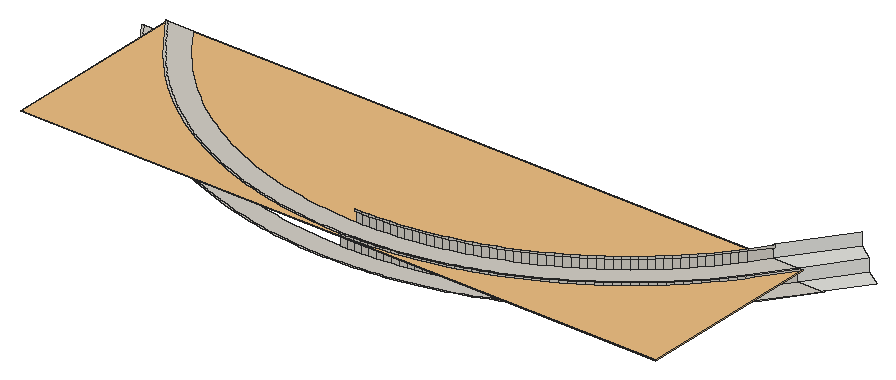
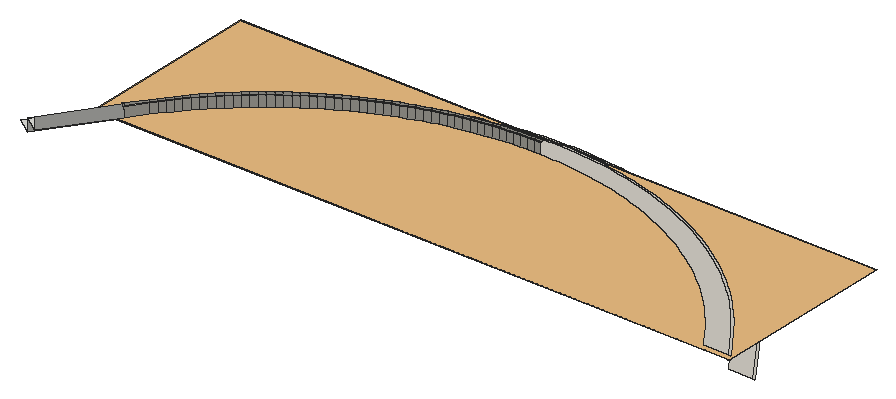
# SketchUp Ruby script. Lengths in inches.
U = 1.inch
M = Sketchup.active_model
def pt(a) = Geom::Point3d.new(a.map { |v| v * U })
def face(e, loops, mat)
  f = e.add_face(loops[0].map { |a| pt(a) })
  loops[1..].each { |l| e.add_face(l.map { |a| pt(a) }).erase! }
  f.material = f.back_material = mat if mat
  f
end
# faces: each face lists its corners as indices into pts; further lists are holes
def faces(e, pts, list, mat = nil) = list.each { |f| face(e, (f[0].is_a?(Array) ? f : [f]).map { |l| l.map { |i| pts[i] } }, mat) }
# xy, xz, yz: faces in a plane at the given z, y or x. An outline is a flat list of corners, or four numbers for a rectangle; further outlines are holes
def ring(l) = l.size == 4 ? [[l[0], l[1]], [l[2], l[1]], [l[2], l[3]], [l[0], l[3]]] : l.each_slice(2).to_a
def flat(e, list, mat, &to3) = list.each { |f| face(e, (f[0].is_a?(Array) ? f : [f]).map { |l| ring(l).map { |u, v| to3.(u, v) } }, mat) }
def xy(e, z, list, mat = nil) = flat(e, list, mat) { |x, y| [x, y, z] }
def xz(e, y, list, mat = nil) = flat(e, list, mat) { |x, z| [x, y, z] }
def yz(e, x, list, mat = nil) = flat(e, list, mat) { |y, z| [x, y, z] }
def lines(e, pts, list) = list.each { |a, b| e.add_line(pt(pts[a]), pt(pts[b])) }
# prism: a flat outline (further loops are holes) pulled along v
def prism(e, loops, v, mat = nil)
  f = face(e, loops, mat); d = Geom::Vector3d.new(v.map { |x| x * U })
  f.pushpull(f.normal.samedirection?(d) ? d.length : -d.length)
end
def box(e, o, s, mat = nil) = prism(e, [[o, [o[0] + s[0], o[1], o[2]], [o[0] + s[0], o[1] + s[1], o[2]], [o[0], o[1] + s[1], o[2]]]], [0, 0, s[2]], mat)
def at(x, y, z, deg = 0) = Geom::Transformation.translation(pt([x, y, z])) * Geom::Transformation.rotation(ORIGIN, Z_AXIS, deg.degrees)
def axes(o, x, y, z) = Geom::Transformation.new([*x, 0, *y, 0, *z, 0, *pt(o).to_a, 1])
def part(name) = M.definitions.add(name)
# library, detail: a bought-in or finely detailed component or shape, given as its bounding box
def library(name, o, s) = part(name).tap { |d| box(d.entities, o, s) }
def detail(e, o, s) = box(e.add_group.entities, o, s)
def put(e, d, t, mat = nil) = e.add_instance(d, t).tap { |i| i.material = mat if mat }
def group(e, t, mat = nil) = e.add_group.tap { |g| g.transformation = t; g.material = mat if mat }.entities
root = M.entities
M.materials.add("Arta-Ceramic-Moonstone-White-24x24-4K").color = [209, 205, 196]
c1 = library("Mesh Light\#6",[-0.5,-0.5,-0.1],[1,1,0.2])
xy(root,18,[[1176.72,194.875,1188.72,194.875,1189.08,195.38,1200.97,212,1193.03,217.67]])
xy(root,18,[[1024.28,97.97,1027.87,98,1031.45,98.11,1035.04,98.28,1038.61,98.52,1042.1875,98.83,1045.76,99.21,1049.3125,99.65,1052.86,100.17,1056.4,100.75,1059.93,101.4,1063.45,102.12,1066.95,102.9,1070.43,103.76,1073.9,104.67,1077.35,105.66,1080.78,106.71,1084.18,107.83,1087.57,109.01,1090.93,110.26,1094.27,111.57,1097.59,112.94,1100.87,114.38,1104.13,115.88,1107.36,117.44,1110.56,119.07,1113.72,120.75,1116.86,122.5,1119.95,124.31,1123.02,126.17,1126.05,128.09,1129.04,130.08,1131.99,132.11,1134.9,134.21,1137.77,136.36,1140.6,138.5625,1143.39,140.82,1146.13,143.13,1148.83,145.5,1151.48,147.91,1154.08,150.38,1156.64,152.89,1159.15,155.46,1161.61,158.07,1164.02,160.73,1166.375,163.43,1168.68,166.18,1170.93,168.97,1173.13,171.81,1175.27,174.68,1189.74,194.91,1189.08,195.38,1188.72,194.875,1174.61,175.16,1172.48,172.3,1170.29,169.48,1168.05,166.7,1165.76,163.96,1163.41,161.27,1161.01,158.62,1158.5625,156.02,1156.07,153.47,1153.52,150.96,1150.93,148.51,1148.29,146.1,1145.6,143.75,1142.87,141.45,1140.09,139.2,1137.28,137.01,1134.42,134.86,1131.52,132.78,1128.58,130.75,1125.6,128.78,1122.59,126.86,1119.54,125,1116.45,123.21,1113.33,121.47,1110.18,119.79,1107,118.17,1103.78,116.62,1100.54,115.12,1097.27,113.69,1093.97,112.32,1090.64,111.02,1087.3,109.77,1083.92,108.6,1080.53,107.49,1077.12,106.4375,1073.68,105.46,1070.23,104.54,1066.76,103.7,1063.28,102.91,1059.78,102.2,1056.26,101.55,1052.74,100.97,1049.21,100.46,1045.66,100.02,1042.11,99.64,1038.55,99.33,1034.99,99.09,1031.42,98.92,1027.85,98.82,1024.28,98.78,1020.71,98.82,1017.14,98.92,1013.57,99.09,1010.01,99.33,1006.45,99.64,1002.9,100.02,999.36,100.46,995.82,100.97,992.3,101.55,988.79,102.2,985.29,102.91,981.8,103.7,978.33,104.54,974.88,105.46,971.45,106.4375,968.03,107.49,964.64,108.6,961.27,109.77,957.92,111.02,954.59,112.32,951.29,113.69,948.02,115.12,944.78,116.62,941.56,118.17,938.38,119.79,935.23,121.47,932.11,123.21,929.02,125,925.97,126.86,922.96,128.78,919.98,130.75,917.04,132.78,914.14,134.86,911.28,137.01,908.47,139.2,905.69,141.45,902.96,143.75,900.28,146.1,897.64,148.51,895.04,150.96,892.5,153.47,890,156.02,887.55,158.62,885.15,161.27,882.81,163.96,880.51,166.7,878.27,169.48,876.08,172.3,873.95,175.16,859.84,194.875,858.84,194.875,873.29,174.68,875.43,171.81,877.63,168.97,879.88,166.18,882.1875,163.43,884.54,160.73,886.95,158.07,889.41,155.46,891.92,152.89,894.48,150.38,897.08,147.91,899.73,145.5,902.43,143.13,905.18,140.82,907.96,138.5625,910.79,136.36,913.66,134.21,916.57,132.11,919.53,130.08,922.52,128.09,925.54,126.17,928.61,124.31,931.71,122.5,934.84,120.75,938.01,119.07,941.2,117.44,944.43,115.88,947.69,114.38,950.98,112.94,954.29,111.57,957.63,110.26,960.99,109.01,964.38,107.83,967.79,106.71,971.22,105.66,974.66,104.67,978.13,103.76,981.62,102.9,985.12,102.12,988.63,101.4,992.16,100.75,995.7,100.17,999.25,99.65,1002.81,99.21,1006.375,98.83,1009.95,98.52,1013.53,98.28,1017.11,98.11,1020.69,98],[1024.28,98.78,1027.85,98.82,1031.42,98.92,1034.99,99.09,1038.55,99.33,1042.11,99.64,1045.66,100.02,1049.21,100.46,1052.74,100.97,1056.26,101.55,1059.78,102.2,1063.28,102.91,1066.76,103.7,1070.23,104.54,1073.68,105.46,1077.12,106.4375,1080.53,107.49,1083.92,108.6,1087.3,109.77,1090.64,111.02,1093.97,112.32,1097.27,113.69,1100.54,115.12,1103.78,116.62,1107,118.17,1110.18,119.79,1113.33,121.47,1116.45,123.21,1119.54,125,1122.59,126.86,1125.6,128.78,1128.58,130.75,1131.52,132.78,1134.42,134.86,1137.28,137.01,1140.09,139.2,1142.87,141.45,1145.6,143.75,1148.29,146.1,1150.93,148.51,1153.52,150.96,1156.07,153.47,1158.5625,156.02,1161.01,158.62,1163.41,161.27,1165.76,163.96,1168.05,166.7,1170.29,169.48,1172.48,172.3,1174.61,175.16,1188.72,194.875,1176.72,194.875,1166.73,180.92,1164.71,178.2,1162.64,175.53,1160.51,172.89,1158.34,170.3,1156.11,167.75,1153.84,165.24,1151.52,162.78,1149.16,160.36,1146.74,157.99,1144.29,155.66,1141.78,153.38,1139.24,151.15,1136.65,148.97,1134.02,146.84,1131.35,144.76,1128.64,142.73,1125.9,140.76,1123.11,138.83,1120.29,136.96,1117.43,135.15,1114.54,133.39,1111.62,131.6875,1108.66,130.04,1105.68,128.45,1102.66,126.92,1099.61,125.44,1096.54,124.02,1093.44,122.67,1090.31,121.37,1087.16,120.13,1083.99,118.96,1080.8,117.84,1077.58,116.79,1074.34,115.8,1071.09,114.87,1067.82,114,1064.53,113.2,1061.23,112.46,1057.91,111.78,1054.59,111.17,1051.25,110.62,1047.9,110.13,1044.54,109.71,1041.18,109.35,1037.8,109.0625,1034.43,108.84,1031.05,108.67,1027.66,108.58,1024.28,108.54,1020.9,108.58,1017.51,108.67,1014.13,108.84,1010.76,109.0625,1007.39,109.35,1004.02,109.71,1000.66,110.13,997.3125,110.62,993.97,111.17,990.65,111.78,987.33,112.46,984.03,113.2,980.74,114,977.47,114.87,974.22,115.8,970.98,116.79,967.77,117.84,964.57,118.96,961.4,120.13,958.25,121.37,955.12,122.67,952.02,124.02,948.95,125.44,945.9,126.92,942.88,128.45,939.9,130.04,936.94,131.6875,934.02,133.39,931.13,135.15,928.27,136.96,925.45,138.83,922.67,140.76,919.92,142.73,917.21,144.76,914.54,146.84,911.91,148.97,909.32,151.15,906.78,153.38,904.28,155.66,901.82,157.99,899.41,160.36,897.04,162.78,894.72,165.24,892.45,167.75,890.22,170.3,888.05,172.89,885.92,175.53,883.85,178.2,881.83,180.92,871.84,194.875,859.84,194.875,873.95,175.16,876.08,172.3,878.27,169.48,880.51,166.7,882.81,163.96,885.15,161.27,887.55,158.62,890,156.02,892.5,153.47,895.04,150.96,897.64,148.51,900.28,146.1,902.96,143.75,905.69,141.45,908.47,139.2,911.28,137.01,914.14,134.86,917.04,132.78,919.98,130.75,922.96,128.78,925.97,126.86,929.02,125,932.11,123.21,935.23,121.47,938.38,119.79,941.56,118.17,944.78,116.62,948.02,115.12,951.29,113.69,954.59,112.32,957.92,111.02,961.27,109.77,964.64,108.6,968.03,107.49,971.45,106.4375,974.88,105.46,978.33,104.54,981.8,103.7,985.29,102.91,988.79,102.2,992.3,101.55,995.82,100.97,999.36,100.46,1002.9,100.02,1006.45,99.64,1010.01,99.33,1013.57,99.09,1017.14,98.92,1020.71,98.82]],"Arta-Ceramic-Moonstone-White-24x24-4K")
xy(root,24,[[1164.72,194.875,1176.72,194.875,1177.08,195.38,1193.03,217.67,1185.09,223.35]])
xy(root,24,[[1024.28,107.73,1027.68,107.76,1031.08,107.86,1034.47,108.02,1037.87,108.25,1041.25,108.54,1044.63,108.9,1048.01,109.33,1051.37,109.8125,1054.73,110.37,1058.07,110.98,1061.4,111.66,1064.72,112.41,1068.02,113.21,1071.31,114.08,1074.58,115.02,1077.83,116.01,1081.06,117.07,1084.27,118.19,1087.45,119.375,1090.62,120.62,1093.76,121.92,1096.875,123.28,1099.96,124.71,1103.02,126.1875,1106.05,127.73,1109.05,129.32,1112.02,130.98,1114.96,132.69,1117.86,134.46,1120.73,136.28,1123.57,138.16,1126.36,140.09,1129.125,142.08,1131.85,144.11,1134.53,146.2,1137.17,148.34,1139.77,150.54,1142.33,152.78,1144.84,155.07,1147.31,157.4,1149.73,159.79,1152.11,162.22,1154.44,164.69,1156.72,167.21,1158.96,169.77,1161.14,172.38,1163.28,175.02,1165.36,177.71,1167.39,180.4375,1177.74,194.91,1177.08,195.38,1176.72,194.875,1166.73,180.92,1164.71,178.2,1162.64,175.53,1160.51,172.89,1158.34,170.3,1156.11,167.75,1153.84,165.24,1151.52,162.78,1149.16,160.36,1146.74,157.99,1144.29,155.66,1141.78,153.38,1139.24,151.15,1136.65,148.97,1134.02,146.84,1131.35,144.76,1128.64,142.73,1125.9,140.76,1123.11,138.83,1120.29,136.96,1117.43,135.15,1114.54,133.39,1111.62,131.6875,1108.66,130.04,1105.68,128.45,1102.66,126.92,1099.61,125.44,1096.54,124.02,1093.44,122.67,1090.31,121.37,1087.16,120.13,1083.99,118.96,1080.8,117.84,1077.58,116.79,1074.34,115.8,1071.09,114.87,1067.82,114,1064.53,113.2,1061.23,112.46,1057.91,111.78,1054.59,111.17,1051.25,110.62,1047.9,110.13,1044.54,109.71,1041.18,109.35,1037.8,109.0625,1034.43,108.84,1031.05,108.67,1027.66,108.58,1024.28,108.54,1020.9,108.58,1017.51,108.67,1014.13,108.84,1010.76,109.0625,1007.39,109.35,1004.02,109.71,1000.66,110.13,997.3125,110.62,993.97,111.17,990.65,111.78,987.33,112.46,984.03,113.2,980.74,114,977.47,114.87,974.22,115.8,970.98,116.79,967.77,117.84,964.57,118.96,961.4,120.13,958.25,121.37,955.12,122.67,952.02,124.02,948.95,125.44,945.9,126.92,942.88,128.45,939.9,130.04,936.94,131.6875,934.02,133.39,931.13,135.15,928.27,136.96,925.45,138.83,922.67,140.76,919.92,142.73,917.21,144.76,914.54,146.84,911.91,148.97,909.32,151.15,906.78,153.38,904.28,155.66,901.82,157.99,899.41,160.36,897.04,162.78,894.72,165.24,892.45,167.75,890.22,170.3,888.05,172.89,885.92,175.53,883.85,178.2,881.83,180.92,871.84,194.875,870.84,194.875,881.17,180.4375,883.2,177.71,885.29,175.02,887.42,172.38,889.61,169.77,891.84,167.21,894.12,164.69,896.45,162.22,898.83,159.79,901.25,157.4,903.72,155.07,906.24,152.78,908.79,150.54,911.39,148.34,914.03,146.2,916.72,144.11,919.4375,142.08,922.2,140.09,924.99,138.16,927.83,136.28,930.7,134.46,933.6,132.69,936.54,130.98,939.51,129.32,942.51,127.73,945.54,126.1875,948.6,124.71,951.6875,123.28,954.8,121.92,957.94,120.62,961.11,119.375,964.29,118.19,967.5,117.07,970.74,116.01,973.99,115.02,977.25,114.08,980.54,113.21,983.84,112.41,987.16,111.66,990.49,110.98,993.84,110.37,997.19,109.8125,1000.55,109.33,1003.93,108.9,1007.31,108.54,1010.7,108.25,1014.09,108.02,1017.48,107.86,1020.88,107.76],[1024.28,108.54,1027.66,108.58,1031.05,108.67,1034.43,108.84,1037.8,109.0625,1041.18,109.35,1044.54,109.71,1047.9,110.13,1051.25,110.62,1054.59,111.17,1057.91,111.78,1061.23,112.46,1064.53,113.2,1067.82,114,1071.09,114.87,1074.34,115.8,1077.58,116.79,1080.8,117.84,1083.99,118.96,1087.16,120.13,1090.31,121.37,1093.44,122.67,1096.54,124.02,1099.61,125.44,1102.66,126.92,1105.68,128.45,1108.66,130.04,1111.62,131.6875,1114.54,133.39,1117.43,135.15,1120.29,136.96,1123.11,138.83,1125.9,140.76,1128.64,142.73,1131.35,144.76,1134.02,146.84,1136.65,148.97,1139.24,151.15,1141.78,153.38,1144.29,155.66,1146.74,157.99,1149.16,160.36,1151.52,162.78,1153.84,165.24,1156.11,167.75,1158.34,170.3,1160.51,172.89,1162.64,175.53,1164.71,178.2,1166.73,180.92,1176.72,194.875,1164.72,194.875,1158.85,186.67,1156.94,184.11,1154.98,181.58,1152.97,179.09,1150.92,176.64,1148.82,174.23,1146.67,171.87,1144.48,169.54,1142.25,167.25,1139.97,165.01,1137.64,162.8125,1135.28,160.66,1132.875,158.55,1130.43,156.49,1127.95,154.48,1125.43,152.52,1122.87,150.6,1120.27,148.73,1117.64,146.92,1114.98,145.15,1112.28,143.4375,1109.55,141.77,1106.79,140.16,1103.99,138.61,1101.17,137.11,1098.32,135.66,1095.45,134.27,1092.54,132.93,1089.61,131.65,1086.66,130.42,1083.68,129.25,1080.6875,128.14,1077.67,127.09,1074.63,126.09,1071.57,125.16,1068.5,124.28,1065.41,123.46,1062.31,122.7,1059.1875,122,1056.05,121.36,1052.91,120.78,1049.76,120.26,1046.59,119.8,1043.42,119.41,1040.24,119.07,1037.06,118.79,1033.87,118.58,1030.67,118.43,1027.48,118.33,1024.28,118.3,1021.08,118.33,1017.89,118.43,1014.7,118.58,1011.51,118.79,1008.32,119.07,1005.14,119.41,1001.97,119.8,998.81,120.26,995.65,120.78,992.51,121.36,989.375,122,986.26,122.7,983.15,123.46,980.0625,124.28,976.99,125.16,973.93,126.09,970.89,127.09,967.875,128.14,964.875,129.25,961.9,130.42,958.95,131.65,956.02,132.93,953.12,134.27,950.24,135.66,947.39,137.11,944.57,138.61,941.77,140.16,939.01,141.77,936.28,143.4375,933.58,145.15,930.92,146.92,928.29,148.73,925.69,150.6,923.13,152.52,920.61,154.48,918.13,156.49,915.68,158.55,913.28,160.66,910.92,162.8125,908.59,165.01,906.32,167.25,904.08,169.54,901.89,171.87,899.74,174.23,897.64,176.64,895.59,179.09,893.58,181.58,891.62,184.11,889.71,186.67,883.84,194.875,871.84,194.875,881.83,180.92,883.85,178.2,885.92,175.53,888.05,172.89,890.22,170.3,892.45,167.75,894.72,165.24,897.04,162.78,899.41,160.36,901.82,157.99,904.28,155.66,906.78,153.38,909.32,151.15,911.91,148.97,914.54,146.84,917.21,144.76,919.92,142.73,922.67,140.76,925.45,138.83,928.27,136.96,931.13,135.15,934.02,133.39,936.94,131.6875,939.9,130.04,942.88,128.45,945.9,126.92,948.95,125.44,952.02,124.02,955.12,122.67,958.25,121.37,961.4,120.13,964.57,118.96,967.77,117.84,970.98,116.79,974.22,115.8,977.47,114.87,980.74,114,984.03,113.2,987.33,112.46,990.65,111.78,993.97,111.17,997.3125,110.62,1000.66,110.13,1004.02,109.71,1007.39,109.35,1010.76,109.0625,1014.13,108.84,1017.51,108.67,1020.9,108.58]],"Arta-Ceramic-Moonstone-White-24x24-4K")
p = [[1024.28,108.54,23],[1024.28,108.54,18],[1027.66,108.58,18],[1027.66,108.58,23],[1031.05,108.67,18],[1031.05,108.67,23],
  [1034.43,108.84,18],[1034.43,108.84,23],[1037.8,109.0625,18],[1037.8,109.0625,23],[1041.18,109.35,18],[1041.18,109.35,23],
  [1044.54,109.71,18],[1044.54,109.71,23],[1047.9,110.13,18],[1047.9,110.13,23],[1051.25,110.62,18],[1051.25,110.62,23],
  [1054.59,111.17,18],[1054.59,111.17,23],[1057.91,111.78,18],[1057.91,111.78,23],[1061.23,112.46,18],[1061.23,112.46,23],
  [1064.53,113.2,18],[1064.53,113.2,23],[1067.82,114,18],[1067.82,114,23],[1071.09,114.87,18],[1071.09,114.87,23],
  [1074.34,115.8,18],[1074.34,115.8,23],[1077.58,116.79,18],[1077.58,116.79,23],[1080.8,117.84,18],[1080.8,117.84,23],
  [1083.99,118.96,18],[1083.99,118.96,23],[1087.16,120.13,18],[1087.16,120.13,23],[1090.31,121.37,18],[1090.31,121.37,23],
  [1093.44,122.67,18],[1093.44,122.67,23],[1096.54,124.02,18],[1096.54,124.02,23],[1099.61,125.44,18],[1099.61,125.44,23],
  [1102.66,126.92,18],[1102.66,126.92,23],[1105.68,128.45,18],[1105.68,128.45,23],[1108.66,130.04,18],[1108.66,130.04,23],
  [1111.62,131.6875,18],[1111.62,131.6875,23],[1114.54,133.39,18],[1114.54,133.39,23],[1117.43,135.15,18],[1117.43,135.15,23],
  [1120.29,136.96,18],[1120.29,136.96,23],[1123.11,138.83,18],[1123.11,138.83,23],[1125.9,140.76,18],[1125.9,140.76,23],
  [1128.64,142.73,18],[1128.64,142.73,23],[1131.35,144.76,18],[1131.35,144.76,23],[1134.02,146.84,18],[1134.02,146.84,23],
  [1136.65,148.97,18],[1136.65,148.97,23],[1139.24,151.15,18],[1139.24,151.15,23],[1141.78,153.38,18],[1141.78,153.38,23],
  [1144.29,155.66,18],[1144.29,155.66,23],[1146.74,157.99,18],[1146.74,157.99,23],[1149.16,160.36,18],[1149.16,160.36,23],
  [1151.52,162.78,18],[1151.52,162.78,23],[1153.84,165.24,18],[1153.84,165.24,23],[1156.11,167.75,18],[1156.11,167.75,23],
  [1158.34,170.3,18],[1158.34,170.3,23],[1160.51,172.89,18],[1160.51,172.89,23],[1162.64,175.53,18],[1162.64,175.53,23],
  [1164.71,178.2,18],[1164.71,178.2,23],[1166.73,180.92,18],[1166.73,180.92,23],[1176.72,194.875,18],[1176.72,194.875,23],
  [1193.03,217.67,24],[1177.08,195.38,24],[1177.08,195.38,23],[1193.03,217.67,18],[1024.28,107.73,24],[1024.28,107.73,23],
  [1027.68,107.76,23],[1027.68,107.76,24],[1031.08,107.86,23],[1031.08,107.86,24],[1034.47,108.02,23],[1034.47,108.02,24],
  [1037.87,108.25,23],[1037.87,108.25,24],[1041.25,108.54,23],[1041.25,108.54,24],[1044.63,108.9,23],[1044.63,108.9,24],
  [1048.01,109.33,23],[1048.01,109.33,24],[1051.37,109.8125,23],[1051.37,109.8125,24],[1054.73,110.37,23],[1054.73,110.37,24],
  [1058.07,110.98,23],[1058.07,110.98,24],[1061.4,111.66,23],[1061.4,111.66,24],[1064.72,112.41,23],[1064.72,112.41,24],
  [1068.02,113.21,23],[1068.02,113.21,24],[1071.31,114.08,23],[1071.31,114.08,24],[1074.58,115.02,23],[1074.58,115.02,24],
  [1077.83,116.01,23],[1077.83,116.01,24],[1081.06,117.07,23],[1081.06,117.07,24],[1084.27,118.19,23],[1084.27,118.19,24],
  [1087.45,119.375,23],[1087.45,119.375,24],[1090.62,120.62,23],[1090.62,120.62,24],[1093.76,121.92,23],[1093.76,121.92,24],
  [1096.875,123.28,23],[1096.875,123.28,24],[1099.96,124.71,23],[1099.96,124.71,24],[1103.02,126.1875,23],[1103.02,126.1875,24],
  [1106.05,127.73,23],[1106.05,127.73,24],[1109.05,129.32,23],[1109.05,129.32,24],[1112.02,130.98,23],[1112.02,130.98,24],
  [1114.96,132.69,23],[1114.96,132.69,24],[1117.86,134.46,23],[1117.86,134.46,24],[1120.73,136.28,23],[1120.73,136.28,24],
  [1123.57,138.16,23],[1123.57,138.16,24],[1126.36,140.09,23],[1126.36,140.09,24],[1129.125,142.08,23],[1129.125,142.08,24],
  [1131.85,144.11,23],[1131.85,144.11,24],[1134.53,146.2,23],[1134.53,146.2,24],[1137.17,148.34,23],[1137.17,148.34,24],
  [1139.77,150.54,23],[1139.77,150.54,24],[1142.33,152.78,23],[1142.33,152.78,24],[1144.84,155.07,23],[1144.84,155.07,24],
  [1147.31,157.4,23],[1147.31,157.4,24],[1149.73,159.79,23],[1149.73,159.79,24],[1152.11,162.22,23],[1152.11,162.22,24],
  [1154.44,164.69,23],[1154.44,164.69,24],[1156.72,167.21,23],[1156.72,167.21,24],[1158.96,169.77,23],[1158.96,169.77,24],
  [1161.14,172.38,23],[1161.14,172.38,24],[1163.28,175.02,23],[1163.28,175.02,24],[1165.36,177.71,23],[1165.36,177.71,24],
  [1167.39,180.4375,23],[1167.39,180.4375,24],[1177.74,194.91,23],[1177.74,194.91,24],[1176.72,194.875,24],[1024.28,118.3,29],
  [1024.28,118.3,24],[1027.48,118.33,24],[1027.48,118.33,29],[1030.67,118.43,24],[1030.67,118.43,29],[1033.87,118.58,24],
  [1033.87,118.58,29],[1037.06,118.79,24],[1037.06,118.79,29],[1040.24,119.07,24],[1040.24,119.07,29],[1043.42,119.41,24],
  [1043.42,119.41,29],[1046.59,119.8,24],[1046.59,119.8,29],[1049.76,120.26,24],[1049.76,120.26,29],[1052.91,120.78,24],
  [1052.91,120.78,29],[1056.05,121.36,24],[1056.05,121.36,29],[1059.1875,122,24],[1059.1875,122,29],[1062.31,122.7,24],
  [1062.31,122.7,29],[1065.41,123.46,24],[1065.41,123.46,29],[1068.5,124.28,24],[1068.5,124.28,29],[1071.57,125.16,24],
  [1071.57,125.16,29],[1074.63,126.09,24],[1074.63,126.09,29],[1077.67,127.09,24],[1077.67,127.09,29],[1080.6875,128.14,24],
  [1080.6875,128.14,29],[1083.68,129.25,24],[1083.68,129.25,29],[1086.66,130.42,24],[1086.66,130.42,29],[1089.61,131.65,24],
  [1089.61,131.65,29],[1092.54,132.93,24],[1092.54,132.93,29],[1095.45,134.27,24],[1095.45,134.27,29],[1098.32,135.66,24],
  [1098.32,135.66,29],[1101.17,137.11,24],[1101.17,137.11,29],[1103.99,138.61,24],[1103.99,138.61,29],[1106.79,140.16,24],
  [1106.79,140.16,29],[1109.55,141.77,24],[1109.55,141.77,29],[1112.28,143.4375,24],[1112.28,143.4375,29],[1114.98,145.15,24],
  [1114.98,145.15,29],[1117.64,146.92,24],[1117.64,146.92,29],[1120.27,148.73,24],[1120.27,148.73,29],[1122.87,150.6,24],
  [1122.87,150.6,29],[1125.43,152.52,24],[1125.43,152.52,29],[1127.95,154.48,24],[1127.95,154.48,29],[1130.43,156.49,24],
  [1130.43,156.49,29],[1132.875,158.55,24],[1132.875,158.55,29],[1135.28,160.66,24],[1135.28,160.66,29],[1137.64,162.8125,24],
  [1137.64,162.8125,29],[1139.97,165.01,24],[1139.97,165.01,29],[1142.25,167.25,24],[1142.25,167.25,29],[1144.48,169.54,24],
  [1144.48,169.54,29],[1146.67,171.87,24],[1146.67,171.87,29],[1148.82,174.23,24],[1148.82,174.23,29],[1150.92,176.64,24],
  [1150.92,176.64,29],[1152.97,179.09,24],[1152.97,179.09,29],[1154.98,181.58,24],[1154.98,181.58,29],[1156.94,184.11,24],
  [1156.94,184.11,29],[1158.85,186.67,24],[1158.85,186.67,29],[1164.72,194.875,24],[1164.72,194.875,29],[1185.09,223.35,30],
  [1165.05,195.33,30],[1165.05,195.33,29],[1185.09,223.35,24],[1024.28,117.49,30],[1024.28,117.49,29],[1027.49,117.52,29],
  [1027.49,117.52,30],[1030.7,117.61,29],[1030.7,117.61,30],[1033.91,117.77,29],[1033.91,117.77,30],[1037.12,117.98,29],
  [1037.12,117.98,30],[1040.32,118.26,29],[1040.32,118.26,30],[1043.51,118.6,29],[1043.51,118.6,30],[1046.7,119,29],
  [1046.7,119,30],[1049.88,119.46,29],[1049.88,119.46,30],[1053.05,119.98,29],[1053.05,119.98,30],[1056.21,120.5625,29],
  [1056.21,120.5625,30],[1059.36,121.2,29],[1059.36,121.2,30],[1062.49,121.91,29],[1062.49,121.91,30],[1065.61,122.67,29],
  [1065.61,122.67,30],[1068.72,123.49,29],[1068.72,123.49,30],[1071.81,124.375,29],[1071.81,124.375,30],[1074.875,125.32,29],
  [1074.875,125.32,30],[1077.93,126.32,29],[1077.93,126.32,30],[1080.96,127.375,29],[1080.96,127.375,30],[1083.97,128.49,29],
  [1083.97,128.49,30],[1086.97,129.67,29],[1086.97,129.67,30],[1089.93,130.9,29],[1089.93,130.9,30],[1092.875,132.1875,29],
  [1092.875,132.1875,30],[1095.79,133.53,29],[1095.79,133.53,30],[1098.68,134.93,29],[1098.68,134.93,30],[1101.55,136.38,29],
  [1101.55,136.38,30],[1104.38,137.89,29],[1104.38,137.89,30],[1107.19,139.46,29],[1107.19,139.46,30],[1109.97,141.08,29],
  [1109.97,141.08,30],[1112.71,142.75,29],[1112.71,142.75,30],[1115.42,144.47,29],[1115.42,144.47,30],[1118.1,146.24,29],
  [1118.1,146.24,30],[1120.74,148.07,29],[1120.74,148.07,30],[1123.35,149.94,29],[1123.35,149.94,30],[1125.92,151.87,29],
  [1125.92,151.87,30],[1128.46,153.84,29],[1128.46,153.84,30],[1130.95,155.87,29],[1130.95,155.87,30],[1133.41,157.9375,29],
  [1133.41,157.9375,30],[1135.82,160.05,29],[1135.82,160.05,30],[1138.2,162.22,29],[1138.2,162.22,30],[1140.53,164.43,29],
  [1140.53,164.43,30],[1142.82,166.68,29],[1142.82,166.68,30],[1145.07,168.97,29],[1145.07,168.97,30],[1147.27,171.3125,29],
  [1147.27,171.3125,30],[1149.43,173.69,29],[1149.43,173.69,30],[1151.54,176.12,29],[1151.54,176.12,30],[1153.6,178.58,29],
  [1153.6,178.58,30],[1155.62,181.08,29],[1155.62,181.08,30],[1157.59,183.62,29],[1157.59,183.62,30],[1159.51,186.19,29],
  [1159.51,186.19,30],[1165.71,194.86,29],[1165.71,194.86,30],[1164.72,194.875,30],[1165.69,194.875,30]]
faces(root,p,[[0,1,2,3],[3,2,4,5],[5,4,6,7],[7,6,8,9],[9,8,10,11],[11,10,12,13],[13,12,14,15],[15,14,16,17],
  [17,16,18,19],[19,18,20,21],[21,20,22,23],[23,22,24,25],[25,24,26,27],[27,26,28,29],[29,28,30,31],[31,30,32,33],
  [33,32,34,35],[35,34,36,37],[37,36,38,39],[39,38,40,41],[41,40,42,43],[43,42,44,45],[45,44,46,47],[47,46,48,49],
  [49,48,50,51],[51,50,52,53],[53,52,54,55],[55,54,56,57],[57,56,58,59],[59,58,60,61],[61,60,62,63],[63,62,64,65],
  [65,64,66,67],[67,66,68,69],[69,68,70,71],[71,70,72,73],[73,72,74,75],[75,74,76,77],[77,76,78,79],[79,78,80,81],
  [81,80,82,83],[83,82,84,85],[85,84,86,87],[87,86,88,89],[89,88,90,91],[91,90,92,93],[93,92,94,95],[95,94,96,97],
  [97,96,98,99],[98,100,101,99],[106,107,108,109],[109,108,110,111],[111,110,112,113],[113,112,114,115],[115,114,116,117],[117,116,118,119],
  [119,118,120,121],[121,120,122,123],[123,122,124,125],[125,124,126,127],[127,126,128,129],[129,128,130,131],[131,130,132,133],[133,132,134,135],
  [135,134,136,137],[137,136,138,139],[139,138,140,141],[141,140,142,143],[143,142,144,145],[145,144,146,147],[147,146,148,149],[149,148,150,151],
  [151,150,152,153],[153,152,154,155],[155,154,156,157],[157,156,158,159],[159,158,160,161],[161,160,162,163],[163,162,164,165],[165,164,166,167],
  [167,166,168,169],[169,168,170,171],[171,170,172,173],[173,172,174,175],[175,174,176,177],[177,176,178,179],[179,178,180,181],[181,180,182,183],
  [183,182,184,185],[185,184,186,187],[187,186,188,189],[189,188,190,191],[191,190,192,193],[193,192,194,195],[195,194,196,197],[197,196,198,199],
  [199,198,200,201],[201,200,202,203],[203,202,204,205],[205,204,206,207],[208,101,104,103],[206,104,103,207],[209,210,211,212],[212,211,213,214],
  [214,213,215,216],[216,215,217,218],[218,217,219,220],[220,219,221,222],[222,221,223,224],[224,223,225,226],[226,225,227,228],[228,227,229,230],
  [230,229,231,232],[232,231,233,234],[234,233,235,236],[236,235,237,238],[238,237,239,240],[240,239,241,242],[242,241,243,244],[244,243,245,246],
  [246,245,247,248],[248,247,249,250],[250,249,251,252],[252,251,253,254],[254,253,255,256],[256,255,257,258],[258,257,259,260],[260,259,261,262],
  [262,261,263,264],[264,263,265,266],[266,265,267,268],[268,267,269,270],[270,269,271,272],[272,271,273,274],[274,273,275,276],[276,275,277,278],
  [278,277,279,280],[280,279,281,282],[282,281,283,284],[284,283,285,286],[286,285,287,288],[288,287,289,290],[290,289,291,292],[292,291,293,294],
  [294,293,295,296],[296,295,297,298],[298,297,299,300],[300,299,301,302],[302,301,303,304],[304,303,305,306],[306,305,307,308],[307,309,310,308],
  [315,316,317,318],[318,317,319,320],[320,319,321,322],[322,321,323,324],[324,323,325,326],[326,325,327,328],[328,327,329,330],[330,329,331,332],
  [332,331,333,334],[334,333,335,336],[336,335,337,338],[338,337,339,340],[340,339,341,342],[342,341,343,344],[344,343,345,346],[346,345,347,348],
  [348,347,349,350],[350,349,351,352],[352,351,353,354],[354,353,355,356],[356,355,357,358],[358,357,359,360],[360,359,361,362],[362,361,363,364],
  [364,363,365,366],[366,365,367,368],[368,367,369,370],[370,369,371,372],[372,371,373,374],[374,373,375,376],[376,375,377,378],[378,377,379,380],
  [380,379,381,382],[382,381,383,384],[384,383,385,386],[386,385,387,388],[388,387,389,390],[390,389,391,392],[392,391,393,394],[394,393,395,396],
  [396,395,397,398],[398,397,399,400],[400,399,401,402],[402,401,403,404],[404,403,405,406],[406,405,407,408],[408,407,409,410],[410,409,411,412],
  [412,411,413,414],[414,413,415,416],[417,310,313,312],[416,415,313,312,418]],"Arta-Ceramic-Moonstone-White-24x24-4K")
faces(root,p,[[102,103,104,101,100,105],[311,312,313,310,309,314]])
g1 = group(root,at(870.84,107.73,23))
xy(g1,0,[[153.4375,0,150.04,0.03,146.64,0.13,143.24,0.29,139.85,0.52,136.46,0.81,133.08,1.17,129.71,1.6,126.35,2.08,122.99,2.64,119.65,3.25,116.32,3.93,113,4.68,109.7,5.48,106.41,6.35,103.14,7.29,99.89,8.28,96.66,9.34,93.45,10.46,90.26,11.64,87.1,12.89,83.96,14.19,80.84,15.55,77.76,16.98,74.7,18.46,71.67,20,68.67,21.59,65.7,23.25,62.76,24.96,59.85,26.73,56.98,28.55,54.15,30.43,51.35,32.36,48.59,34.35,45.87,36.38,43.19,38.47,40.55,40.62,37.95,42.81,35.39,45.05,32.88,47.34,30.41,49.67,27.99,52.06,25.61,54.49,23.28,56.96,21,59.48,18.76,62.04,16.58,64.65,14.44,67.29,12.36,69.98,10.33,72.71,0,87.15,1,87.15,10.99,73.1875,13.01,70.47,15.08,67.8,17.21,65.16,19.38,62.57,21.6,60.02,23.875,57.51,26.2,55.05,28.5625,52.63,30.98,50.26,33.43,47.93,35.94,45.65,38.48,43.42,41.07,41.24,43.7,39.11,46.37,37.03,49.07,35,51.82,33.03,54.61,31.1,57.43,29.23,60.28,27.42,63.17,25.66,66.1,23.96,69.05,22.31,72.04,20.72,75.06,19.19,78.1,17.71,81.18,16.29,84.28,14.9375,87.4,13.64,90.55,12.4,93.73,11.23,96.92,10.11,100.14,9.06,103.375,8.07,106.63,7.14,109.9,6.27,113.1875,5.47,116.49,4.73,119.8,4.05,123.13,3.4375,126.47,2.89,129.82,2.4,133.18,1.98,136.54,1.625,139.91,1.33,143.29,1.11,146.67,0.94,150.05,0.85,153.4375,0.8125,156.82,0.85,160.2,0.94,163.58,1.11,166.96,1.33,170.33,1.625,173.7,1.98,177.06,2.4,180.4,2.89,183.74,3.4375,187.07,4.05,190.39,4.73,193.6875,5.47,196.98,6.27,200.25,7.14,203.5,8.07,206.74,9.06,209.95,10.11,213.15,11.23,216.32,12.4,219.47,13.64,222.6,14.9375,225.7,16.29,228.77,17.71,231.82,19.19,234.83,20.72,237.82,22.31,240.78,23.96,243.7,25.66,246.59,27.42,249.45,29.23,252.27,31.1,255.05,33.03,257.8,35,260.51,37.03,263.18,39.11,265.81,41.24,268.39,43.42,270.94,45.65,273.44,47.93,275.9,50.26,278.3125,52.63,280.68,55.05,283,57.51,285.27,60.02,287.5,62.57,289.67,65.16,291.79,67.8,293.87,70.47,295.89,73.1875,305.875,87.15,306.24,87.65,306.9,87.18,296.55,72.71,294.51,69.98,292.43,67.29,290.3,64.65,288.11,62.04,285.88,59.48,283.6,56.96,281.27,54.49,278.89,52.06,276.46,49.67,274,47.34,271.48,45.05,268.92,42.81,266.33,40.62,263.68,38.47,261,36.38,258.28,34.35,255.52,32.36,252.72,30.43,249.89,28.55,247.02,26.73,244.12,24.96,241.18,23.25,238.21,21.59,235.21,20,232.18,18.46,229.12,16.98,226.03,15.55,222.92,14.19,219.78,12.89,216.61,11.64,213.42,10.46,210.21,9.34,206.98,8.28,203.73,7.29,200.46,6.35,197.18,5.48,193.875,4.68,190.56,3.93,187.23,3.25,183.88,2.64,180.53,2.08,177.16,1.6,173.79,1.17,170.41,0.81,167.02,0.52,163.63,0.29,160.24,0.13,156.84,0.03]],"Arta-Ceramic-Moonstone-White-24x24-4K")
put(g1,c1,axes([153.45,43.83,0],[307.90009,0,0],[0,88.6535,0],[0,0,1]))
